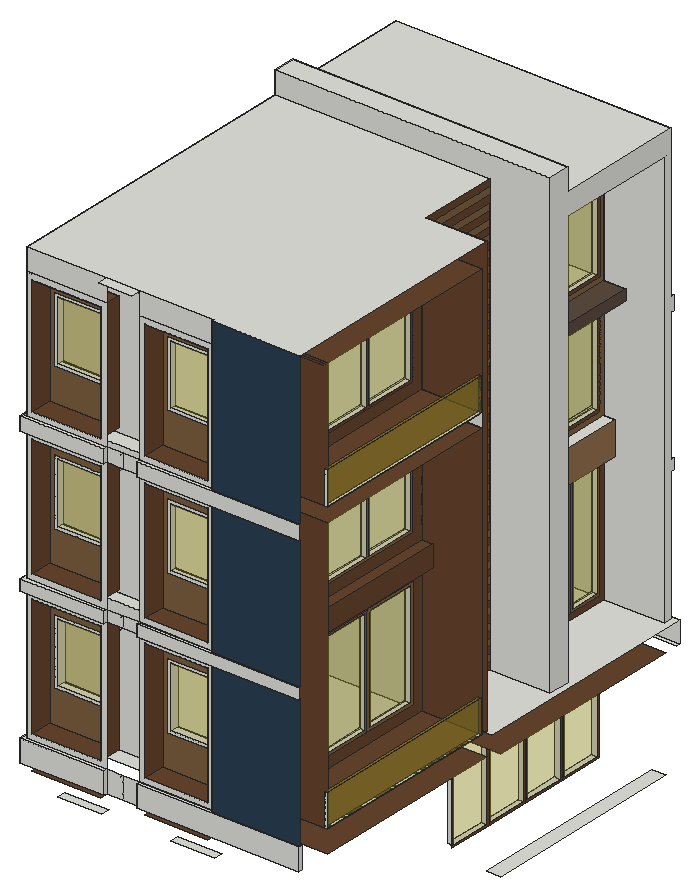
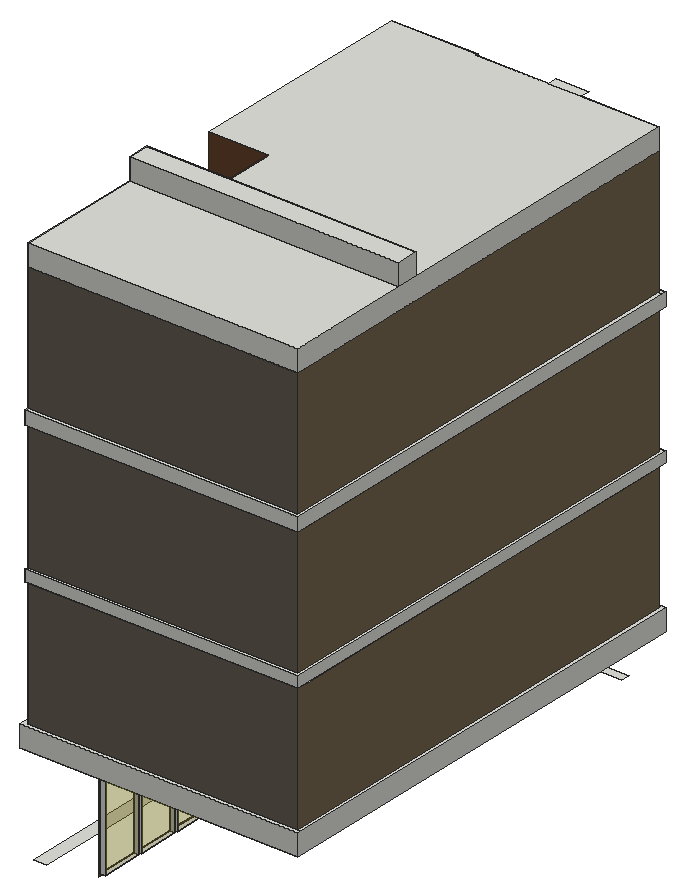
# SketchUp Ruby script. Lengths in inches.
U = 1.inch
M = Sketchup.active_model
def pt(a) = Geom::Point3d.new(a.map { |v| v * U })
def face(e, loops, mat)
  f = e.add_face(loops[0].map { |a| pt(a) })
  loops[1..].each { |l| e.add_face(l.map { |a| pt(a) }).erase! }
  f.material = f.back_material = mat if mat
  f
end
# faces: each face lists its corners as indices into pts; further lists are holes
def faces(e, pts, list, mat = nil) = list.each { |f| face(e, (f[0].is_a?(Array) ? f : [f]).map { |l| l.map { |i| pts[i] } }, mat) }
# xy, xz, yz: faces in a plane at the given z, y or x. An outline is a flat list of corners, or four numbers for a rectangle; further outlines are holes
def ring(l) = l.size == 4 ? [[l[0], l[1]], [l[2], l[1]], [l[2], l[3]], [l[0], l[3]]] : l.each_slice(2).to_a
def flat(e, list, mat, &to3) = list.each { |f| face(e, (f[0].is_a?(Array) ? f : [f]).map { |l| ring(l).map { |u, v| to3.(u, v) } }, mat) }
def xy(e, z, list, mat = nil) = flat(e, list, mat) { |x, y| [x, y, z] }
def xz(e, y, list, mat = nil) = flat(e, list, mat) { |x, z| [x, y, z] }
def yz(e, x, list, mat = nil) = flat(e, list, mat) { |y, z| [x, y, z] }
def lines(e, pts, list) = list.each { |a, b| e.add_line(pt(pts[a]), pt(pts[b])) }
# prism: a flat outline (further loops are holes) pulled along v
def prism(e, loops, v, mat = nil)
  f = face(e, loops, mat); d = Geom::Vector3d.new(v.map { |x| x * U })
  f.pushpull(f.normal.samedirection?(d) ? d.length : -d.length)
end
def box(e, o, s, mat = nil) = prism(e, [[o, [o[0] + s[0], o[1], o[2]], [o[0] + s[0], o[1] + s[1], o[2]], [o[0], o[1] + s[1], o[2]]]], [0, 0, s[2]], mat)
def at(x, y, z, deg = 0) = Geom::Transformation.translation(pt([x, y, z])) * Geom::Transformation.rotation(ORIGIN, Z_AXIS, deg.degrees)
def axes(o, x, y, z) = Geom::Transformation.new([*x, 0, *y, 0, *z, 0, *pt(o).to_a, 1])
def part(name) = M.definitions.add(name)
# library, detail: a bought-in or finely detailed component or shape, given as its bounding box
def library(name, o, s) = part(name).tap { |d| box(d.entities, o, s) }
def detail(e, o, s) = box(e.add_group.entities, o, s)
def put(e, d, t, mat = nil) = e.add_instance(d, t).tap { |i| i.material = mat if mat }
def group(e, t, mat = nil) = e.add_group.tap { |g| g.transformation = t; g.material = mat if mat }.entities
root = M.entities
M.materials.add("Carpet_04_1K").color = [43, 65, 85]
M.materials.add("Glass_Basic_01").color = [186, 175, 42]
M.materials["Glass_Basic_01"].alpha = 0.25
M.materials.add("Glass_Basic_1").color = [186, 174, 38]
M.materials["Glass_Basic_1"].alpha = 0.25
M.materials.add("Plaster_03_1K").color = [121, 105, 83]
M.materials.add("Plaster_04_1K").color = [106, 98, 87]
M.materials.add("Plywood_01_1K").color = [125, 96, 64]
M.materials.add("Wood_Floor_01_1K").color = [146, 111, 76]
M.materials.add("Wood_Floor_12_1K").color = [92, 75, 65]
M.materials.add("Wood_Veneer_15_1K").color = [103, 69, 45]
c1 = part("Group\#1")
xy(c1.entities,0,[[0,0,3,210]])
xy(c1.entities,36,[[0,0,3,210]],"Glass_Basic_01")
xz(c1.entities,0,[[0,0,3,36]])
xz(c1.entities,210,[[0,0,3,36]])
yz(c1.entities,0,[[0,0,210,36]],"Glass_Basic_01")
yz(c1.entities,3,[[0,0,210,36]],"Glass_Basic_01")
c2 = library("Sphere Light\#3",[-2.79,-2.79,-2.79],[5.58,5.58,5.58])
c3 = library("Sphere Light\#2",[-2.6,-2.6,-2.6],[5.2,5.2,5.2])
c4 = library("Sphere Light\#1",[-1.86,-1.86,-1.86],[3.72,3.72,3.72])
c5 = library("Sphere Light",[-2.55,-2.55,-2.55],[5.1,5.1,5.1])
xy(root,60,[[295,274,310,499]])
xy(root,62,[[241,288,247,334.25],[241,338.25,247,384.5],[241,388.5,247,434.75],[241,438.75,247,485]])
xy(root,141,[[19,34,67,43],[142,34,190,43]])
xy(root,165,[[241,49,247,119],[241,122,247,186],[241,189,247,259]])
xy(root,166,[[241,288,247,334.25],[241,338.25,247,384.5],[241,388.5,247,434.75],[241,438.75,247,485]])
xy(root,174,[[10,10,85,34],[133,10,202,34]],"Wood_Veneer_15_1K")
xy(root,180,[[0,6,4,514],[4,6,91,10],[127,6,127,10,208,10,208,8,304,8,304,6],[0,514,310,518]])
xy(root,180,[[208,8,304,10]],"Carpet_04_1K")
xy(root,180,[[247,46,304,262],[247,274,310,499]],"Wood_Veneer_15_1K")
xy(root,192,[[13,43,241,505]])
xy(root,204,[[0,6,4,514],[4,6,91,10],[127,6,304,6,304,8,208,8,208,10,127,10],[13,43,232,256],[238,262,310,262,310,518,0,518,0,514,304,514,304,505,238,505,238,373,304,373,304,349,238,349],
  [13,262,232,505]])
xy(root,204,[[208,8,304,10]],"Carpet_04_1K")
xy(root,204,[[238,46,304,256]],"Wood_Veneer_15_1K")
xy(root,210,[[10,10,85,34],[133,10,202,34]],"Wood_Veneer_15_1K")
xy(root,213,[[232,382,238,416],[232,422,238,456],[232,462,238,496]])
xy(root,219,[[232,61,238,117],[232,123,238,179],[232,185,238,241]])
xy(root,249,[[19,34,73,43],[142,34,196,43]])
xy(root,315,[[19,34,73,43],[142,34,196,43]])
xy(root,333,[[232,61,238,117],[232,123,238,179],[232,185,238,241]])
xy(root,339,[[232,382,238,416],[232,422,238,456],[232,462,238,496]])
xy(root,342,[[10,10,85,34],[133,10,202,34]],"Wood_Veneer_15_1K")
xy(root,348,[[0,6,4,43],[4,6,91,10],[127,6,127,10,208,10,208,8,304,8,304,6],[0,43,4,256],[4,43,13,256],
  [13,43,232,256],[0,256,4,262],[4,256,232,262],[0,262,4,349],[4,262,13,349],
  [13,262,232,505],[0,349,4,373],[4,349,13,373],[238,361,250,373],[0,373,4,505],
  [4,373,13,505],[238,373,250,505],[0,505,4,518],[4,514,304,518]])
xy(root,348,[[238,46,250,256]],"Wood_Veneer_15_1K")
xy(root,360,[[0,6,91,6,91,10,4,10,4,514,304,514,304,518,0,518],[127,6,304,6,304,8,208,8,208,10,127,10],[10,40,232,508]])
xy(root,366,[[10,10,85,34],[133,10,202,34]],"Wood_Veneer_15_1K")
xy(root,372,[[238,361,250,373]])
xy(root,372,[[238,46,250,256]],"Wood_Veneer_15_1K")
xy(root,384,[[238,373,250,505]])
xy(root,387,[[232,61,238,121],[232,124,238,181],[232,184,238,241]])
xy(root,393,[[232,382,238,436],[232,442,238,496]])
xy(root,405,[[19,34,73,40],[142,34,196,40]])
xy(root,471,[[19,34,73,40],[142,34,196,40]])
xy(root,489,[[232,61,238,121],[232,124,238,181],[232,184,238,241]])
xy(root,495,[[232,382,238,436],[232,442,238,496]])
xy(root,498,[[10,10,85,34],[133,10,202,34]],"Wood_Veneer_15_1K")
xy(root,504,[[0,6,91,10],[127,6,127,10,208,10,208,8,304,8,304,6],[0,10,4,508],[10,40,232,508],[232,43,238,46],
  [238,361,262,373],[0,508,4,518],[4,508,238,514],[4,514,238,518],[238,514,304,518]])
xy(root,504,[[238,373,262,505]],"Wood_Floor_12_1K")
xy(root,504,[[[238,46,304,256],[269.9,73.71,270.68,73.8125,271.4,74.11,272.02,74.59,272.5,75.21,272.8,75.93,272.9,76.71,272.8,77.49,272.5,78.21,272.02,78.83,271.4,79.31,270.68,79.61,269.9,79.71,269.125,79.61,268.4,79.31,267.78,78.83,267.3,78.21,267,77.49,266.9,76.71,267,75.93,267.3,75.21,267.78,74.59,268.4,74.11,269.125,73.8125],[269.9,225.375,270.68,225.48,271.4,225.78,272.02,226.26,272.5,226.875,272.8,227.6,272.9,228.375,272.8,229.15,272.5,229.875,272.02,230.5,271.4,230.97,270.68,231.27,269.9,231.375,269.125,231.27,268.4,230.97,267.78,230.5,267.3,229.875,267,229.15,266.9,228.375,267,227.6,267.3,226.875,267.78,226.26,268.4,225.78,269.125,225.48]]],"Wood_Veneer_15_1K")
xy(root,508,[[269.9,73.71,269.125,73.8125,268.4,74.11,267.78,74.59,267.3,75.21,267,75.93,266.9,76.71,267,77.49,267.3,78.21,267.78,78.83,268.4,79.31,269.125,79.61,269.9,79.71,270.68,79.61,271.4,79.31,272.02,78.83,272.5,78.21,272.8,77.49,272.9,76.71,272.8,75.93,272.5,75.21,272.02,74.59,271.4,74.11,270.68,73.8125],[269.9,225.375,269.125,225.48,268.4,225.78,267.78,226.26,267.3,226.875,267,227.6,266.9,228.375,267,229.15,267.3,229.875,267.78,230.5,268.4,230.97,269.125,231.27,269.9,231.375,270.68,231.27,271.4,230.97,272.02,230.5,272.5,229.875,272.8,229.15,272.9,228.375,272.8,227.6,272.5,226.875,272.02,226.26,271.4,225.78,270.68,225.48]],"Wood_Veneer_15_1K")
xy(root,516,[[10,40,232,508],[238,361,262,373]])
xy(root,516,[[238,373,262,505]],"Wood_Floor_12_1K")
xy(root,519,[[0,6,91,10],[127,6,304,6,304,8,208,8,208,10,127,10],[0,10,4,518],[4,514,304,518]])
xy(root,519,[[238,46,304,256]],"Wood_Veneer_15_1K")
xy(root,525,[[232,382,238,436],[232,442,238,496]])
xy(root,525,[[10,10,85,34],[133,10,202,34]],"Wood_Veneer_15_1K")
xy(root,534,[[232,61,238,121],[232,124,238,181],[232,184,238,241]])
xy(root,564,[[19,34,73,40],[142,34,196,40]])
xy(root,627,[[232,382,238,436],[232,442,238,496]])
xy(root,630,[[19,34,73,40],[142,34,196,40]])
xy(root,645,[[232,61,238,121],[232,124,238,181],[232,184,238,241]])
xy(root,654,[[10,10,85,34],[133,10,202,34]],"Wood_Veneer_15_1K")
xy(root,660,[[4,10,10,514],[10,40,232,508],[232,43,238,46],[232,46,238,262],[232,262,238,349],
  [232,349,238,508],[10,508,238,514]])
xy(root,660,[[[238,46,304,256],[269.9,73.71,270.68,73.8125,271.4,74.11,272.02,74.59,272.5,75.21,272.8,75.93,272.9,76.71,272.8,77.49,272.5,78.21,272.02,78.83,271.4,79.31,270.68,79.61,269.9,79.71,269.125,79.61,268.4,79.31,267.78,78.83,267.3,78.21,267,77.49,266.9,76.71,267,75.93,267.3,75.21,267.78,74.59,268.4,74.11,269.125,73.8125],[269.9,225.375,270.68,225.48,271.4,225.78,272.02,226.26,272.5,226.875,272.8,227.6,272.9,228.375,272.8,229.15,272.5,229.875,272.02,230.5,271.4,230.97,270.68,231.27,269.9,231.375,269.125,231.27,268.4,230.97,267.78,230.5,267.3,229.875,267,229.15,266.9,228.375,267,227.6,267.3,226.875,267.78,226.26,268.4,225.78,269.125,225.48]],[238,373,304,505]],"Wood_Veneer_15_1K")
xy(root,664,[[269.9,73.71,269.125,73.8125,268.4,74.11,267.78,74.59,267.3,75.21,267,75.93,266.9,76.71,267,77.49,267.3,78.21,267.78,78.83,268.4,79.31,269.125,79.61,269.9,79.71,270.68,79.61,271.4,79.31,272.02,78.83,272.5,78.21,272.8,77.49,272.9,76.71,272.8,75.93,272.5,75.21,272.02,74.59,271.4,74.11,270.68,73.8125],[269.9,225.375,269.125,225.48,268.4,225.78,267.78,226.26,267.3,226.875,267,227.6,266.9,228.375,267,229.15,267.3,229.875,267.78,230.5,268.4,230.97,269.125,231.27,269.9,231.375,270.68,231.27,271.4,230.97,272.02,230.5,272.5,229.875,272.8,229.15,272.9,228.375,272.8,227.6,272.5,226.875,272.02,226.26,271.4,225.78,270.68,225.48]],"Wood_Veneer_15_1K")
xy(root,684,[[91,0,127,10],[208,8,304,8,304,262,238,262,238,349,4,349,4,10,208,10],[4,373,304,514]])
xy(root,708,[[4,349,304,373]])
xz(root,6,[[0,180,91,204],[127,180,304,204],[0,348,91,360],[127,348,304,360],[0,504,91,519],
  [127,504,304,519]])
xz(root,8,[[208,204,304,348],[208,360,304,504],[208,519,304,684]],"Carpet_04_1K")
xz(root,10,[[91,180,109,204],[109,180,127,204],[127,180,208,204],[208,180,304,204],[[4,204,91,348],[10,210,85,342]],
  [[127,204,208,348],[133,210,202,342]],[91,348,109,360],[109,348,127,360],[127,348,208,360],[[4,360,91,504],[10,366,85,498]],
  [[127,360,208,504],[133,366,202,498]],[91,504,109,519],[109,504,127,519],[127,504,208,519],[[4,519,91,660],[10,525,85,654]],
  [[127,519,208,660],[133,525,202,654]],[4,660,91,684],[127,660,208,684]])
xz(root,34,[[[16,246,76,318],[19,249,73,315]],[[139,246,199,318],[142,249,196,315]],[[16,402,76,474],[19,405,73,471]],[[139,402,199,474],[142,405,196,471]],[[16,561,76,633],[19,564,73,630]],
  [[139,561,199,633],[142,564,196,630]]])
xz(root,34,[[19,249,73,315],[142,249,196,315],[19,405,73,471],[142,405,196,471],[19,564,73,630],
  [142,564,196,630]],"Glass_Basic_1")
xz(root,34,[[[10,210,85,342],[16,246,76,318]],[[133,210,202,342],[139,246,199,318]],[[10,366,85,498],[16,402,76,474]],[[133,366,202,498],[139,402,199,474]],[[10,525,85,654],[16,561,76,633]],
  [[133,525,202,654],[139,561,199,633]]],"Plywood_01_1K")
xz(root,40,[[[10,360,232,504],[19,405,73,471],[142,405,196,471]],[[10,516,232,660],[19,564,73,630],[142,564,196,630]]])
xz(root,40,[[19,405,73,471],[142,405,196,471],[19,564,73,630],[142,564,196,630]],"Glass_Basic_1")
xz(root,43,[[[13,204,232,348],[142,249,196,315],[19,249,73,315]]])
xz(root,43,[[19,249,73,315],[142,249,196,315]],"Glass_Basic_1")
xz(root,46,[[238,348,250,372]])
xz(root,46,[[238,204,238,348,250,348,250,372,238,372,238,504,304,504,304,240,301,240,301,204],[238,519,304,660]],"Wood_Veneer_15_1K")
xz(root,61,[[232,219,238,333],[232,387,238,489],[232,534,238,645]])
xz(root,117,[[232,219,238,333]])
xz(root,121,[[232,387,238,489],[232,534,238,645]])
xz(root,123,[[232,219,238,333]])
xz(root,124,[[232,387,238,489],[232,534,238,645]])
xz(root,179,[[232,219,238,333]])
xz(root,181,[[232,387,238,489],[232,534,238,645]])
xz(root,184,[[232,387,238,489],[232,534,238,645]])
xz(root,185,[[232,219,238,333]])
xz(root,241,[[232,219,238,333],[232,387,238,489],[232,534,238,645]])
xz(root,256,[[13,204,232,348],[238,348,250,360],[238,360,250,372],[238,504,304,519]])
xz(root,256,[[238,204,304,204,304,504,238,504,238,372,250,372,250,348,238,348],[238,519,304,660]],"Wood_Veneer_15_1K")
xz(root,262,[[13,204,232,348]])
xz(root,262,[[238,204,304,684]],"Wood_Veneer_15_1K")
xz(root,288,[[241,62,247,166]])
xz(root,334.25,[[241,62,247,166]])
xz(root,338.25,[[241,62,247,166]])
xz(root,349,[[238,204,304,204,304,708,4,708,4,684,238,684]])
xz(root,361,[[238,348,250,360],[238,360,250,372],[238,504,262,516]])
xz(root,373,[[238,372,250,384],[4,684,304,708]])
xz(root,373,[[238,204,238,348,250,348,250,384,238,384,238,504,262,504,262,516,238,516,238,660,304,660,304,204]],"Wood_Veneer_15_1K")
xz(root,382,[[232,213,238,339],[232,393,238,495],[232,525,238,627]])
xz(root,384.5,[[241,62,247,166]])
xz(root,388.5,[[241,62,247,166]])
xz(root,416,[[232,213,238,339]])
xz(root,422,[[232,213,238,339]])
xz(root,434.75,[[241,62,247,166]])
xz(root,436,[[232,393,238,495],[232,525,238,627]])
xz(root,438.75,[[241,62,247,166]])
xz(root,442,[[232,393,238,495],[232,525,238,627]])
xz(root,456,[[232,213,238,339]])
xz(root,462,[[232,213,238,339]])
xz(root,485,[[241,62,247,166]])
xz(root,496,[[232,213,238,339],[232,393,238,495],[232,525,238,627]])
xz(root,505,[[13,204,232,348],[238,204,304,204,304,660,238,660,238,516,262,516,262,504,238,504,238,384,250,384,250,348,238,348],[238,348,250,360],[238,360,250,384],[238,504,262,516]])
xz(root,508,[[10,360,232,504],[10,516,232,660]])
xz(root,514,[[4,660,304,684]])
xz(root,514,[[4,204,304,348],[4,360,304,504],[4,519,304,660]],"Plaster_04_1K")
xz(root,518,[[0,180,310,204],[0,348,304,360],[0,504,304,519]])
yz(root,0,[[6,180,518,204],[6,348,518,360],[6,504,518,519]])
yz(root,4,[[10,660,514,684],[349,684,373,708]])
yz(root,4,[[10,204,514,348],[10,360,514,504],[10,519,514,660]],"Plaster_03_1K")
yz(root,10,[[40,360,508,504],[40,516,508,660]])
yz(root,10,[[10,210,34,342],[10,366,34,498],[10,525,34,654]],"Wood_Veneer_15_1K")
yz(root,13,[[43,204,256,348],[262,204,505,348]])
yz(root,19,[[34,249,43,315],[34,405,40,471],[34,564,40,630]])
yz(root,73,[[34,249,43,315],[34,405,40,471],[34,564,40,630]])
yz(root,85,[[10,210,34,342],[10,366,34,498],[10,525,34,654]],"Wood_Veneer_15_1K")
yz(root,91,[[6,180,10,204],[6,348,10,360],[6,504,10,519]])
yz(root,127,[[6,180,10,204],[6,348,10,360],[6,504,10,519]])
yz(root,133,[[10,210,34,342],[10,366,34,498],[10,525,34,654]],"Wood_Veneer_15_1K")
yz(root,142,[[34,249,43,315],[34,405,40,471],[34,564,40,630]])
yz(root,196,[[34,249,43,315],[34,405,40,471],[34,564,40,630]])
yz(root,202,[[10,210,34,342],[10,366,34,498],[10,525,34,654]],"Wood_Veneer_15_1K")
yz(root,208,[[8,204,10,348],[8,360,10,504]],"Carpet_04_1K")
yz(root,208,[[8,519,10,660],[8,660,10,684]],"Plaster_04_1K")
yz(root,232,[[[43,204,256,348],[185,219,241,333],[123,219,179,333],[61,219,117,333]],[[262,204,505,348],[382,213,416,339],[422,213,456,339],[462,213,496,339]],[40,360,43,504],[43,360,46,504],[[46,360,508,504],[61,387,121,489],[184,387,241,489],[124,387,181,489],[442,393,496,495],[382,393,436,495]],
  [442,393,496,395.46],[40,516,43,660],[43,516,46,660],[[46,516,508,660],[61,534,121,645],[124,534,181,645],[184,534,241,645],[382,525,436,627],[442,525,496,627]]])
yz(root,232,[[382,213,416,339],[422,213,456,339],[462,213,496,339],[61,219,117,333],[123,219,179,333],
  [185,219,241,333],[61,387,121,489],[124,387,181,489],[184,387,241,489],[382,393,436,495],
  [442,395.46,496,495],[382,525,436,627],[442,525,496,627],[61,534,121,645],[124,534,181,645],
  [184,534,241,645]],"Glass_Basic_01")
yz(root,238,[[43,348,46,504],[256,348,262,360],[349,348,361,360],[256,360,262,504],[349,360,361,360,361,372,373,372,373,504,349,504],
  [43,504,46,660],[256,504,262,516],[349,504,361,516],[505,504,508,516],[256,516,262,660],
  [349,516,373,660],[505,516,508,660]])
yz(root,238,[[382,213,416,339],[422,213,456,339],[462,213,496,339],[61,219,117,333],[123,219,179,333],
  [185,219,241,333],[61,387,121,489],[124,387,181,489],[184,387,241,489],[382,393,436,495],
  [442,393,496,495],[382,525,436,627],[442,525,496,627],[61,534,121,645],[124,534,181,645],
  [184,534,241,645]],"Glass_Basic_01")
yz(root,238,[[[379,210,419,342],[382,213,416,339]],[[419,210,459,342],[422,213,456,339]],[[459,210,499,342],[462,213,496,339]],[262,211.6,349,219.2],[[58,216,120,336],[61,219,117,333]],
  [[120,216,182,336],[123,219,179,333]],[[182,216,244,336],[185,219,241,333]],[262,226.8,349,234.4],[262,242,349,249.6],[262,257.2,349,264.8],
  [262,272.4,349,280],[262,287.6,349,295.2],[262,302.8,349,310.4],[262,318,349,325.6],[262,333.2,349,340.8],
  [262,348.4,349,356],[262,363.6,349,371.2],[262,378.8,349,386.4],[[58,384,244,492],[61,387,61,489,121,489,121,387,124,387,124,489,181,489,181,387,184,387,184,489,241,489,241,387]],[[373,384,505,504],[379,390,499,498]],
  [262,394,349,401.6],[262,409.2,349,416.8],[262,424.4,349,432],[262,439.6,349,447.2],[262,454.8,349,462.4],
  [262,470,349,477.6],[262,485.2,349,492.8],[262,500.4,349,508],[262,515.6,349,523.2],[[373,516,505,636],[379,522,499,630]],
  [262,530.8,349,538.4],[262,546,349,553.6],[262,561.2,349,568.8],[262,576.4,349,584],[262,591.6,349,599.2],
  [262,606.8,349,614.4],[262,622,349,629.6],[262,637.2,349,644.8],[262,652.4,349,660],[262,668,349,676]],"Plywood_01_1K")
yz(root,238,[[373,636,505,660]],"Wood_Floor_01_1K")
yz(root,238,[[[46,204,256,348],[58,216,244,336]],[262,204,349,211.6],[[373,204,505,348],[379,210,499,342]],[262,219.2,349,226.8],[262,234.4,349,242],
  [262,249.6,349,257.2],[262,264.8,349,272.4],[262,280,349,287.6],[262,295.2,349,302.8],[262,310.4,349,318],
  [262,325.6,349,333.2],[262,340.8,349,348.4],[262,356,349,363.6],[262,371.2,349,378.8],[[46,372,256,504],[58,384,244,492]],
  [262,386.4,349,394],[[379,390,439,498],[382,393,436,495]],[[439,390,499,498],[442,393,496,495]],[262,401.6,349,409.2],[262,416.8,349,424.4],
  [262,432,349,439.6],[262,447.2,349,454.8],[262,462.4,349,470],[262,477.6,349,485.2],[262,492.8,349,500.4],
  [262,508,349,515.6],[[46,519,256,660],[58,531,244,648]],[[379,522,439,630],[382,525,436,627]],[[439,522,499,630],[442,525,496,627]],[262,523.2,349,530.8],
  [[58,531,244,648],[61,534,61,645,121,645,121,534,124,534,124,645,181,645,181,534,184,534,184,645,241,645,241,534]],[262,538.4,349,546],[262,553.6,349,561.2],[262,568.8,349,576.4],[262,584,349,591.6],
  [262,599.2,349,606.8],[262,614.4,349,622],[262,629.6,349,637.2],[262,644.8,349,652.4],[262,660,349,668],
  [262,676,349,684]],"Wood_Veneer_15_1K")
yz(root,241,[[288,62,334.25,166],[338.25,62,384.5,166],[388.5,62,434.75,166],[438.75,62,485,166]],"Glass_Basic_01")
yz(root,247,[[288,62,334.25,166],[338.25,62,384.5,166],[388.5,62,434.75,166],[438.75,62,485,166]],"Glass_Basic_01")
yz(root,247,[[[286,60,336.25,168],[288,62,334.25,166]],[[336.25,60,386.5,168],[338.25,62,384.5,166]],[[386.5,60,436.75,168],[388.5,62,434.75,166]],[[436.75,60,487,168],[438.75,62,485,166]]],"Wood_Veneer_15_1K")
yz(root,250,[[361,348,373,360],[361,360,373,372]])
yz(root,250,[[373,348,505,384]],"Wood_Floor_01_1K")
yz(root,250,[[46,348,256,372]],"Wood_Veneer_15_1K")
yz(root,262,[[361,504,373,516]])
yz(root,262,[[373,504,505,516]],"Wood_Floor_12_1K")
yz(root,304,[[6,180,10,204],[349,204,373,204,373,660,505,660,505,204,514,204,514,348,518,348,518,360,514,360,514,504,518,504,518,519,514,519,514,684,373,684,373,708,349,708]])
p = [[269.9,73.71,504],[269.125,73.8125,504],[269.125,73.8125,508],[269.9,73.71,508],[270.68,73.8125,504],[270.68,73.8125,508],
  [268.4,74.11,504],[268.4,74.11,508],[271.4,74.11,504],[271.4,74.11,508],[267.78,74.59,504],[267.78,74.59,508],
  [272.02,74.59,504],[272.02,74.59,508],[267.3,75.21,504],[267.3,75.21,508],[272.5,75.21,504],[272.5,75.21,508],
  [267,75.93,504],[267,75.93,508],[272.8,75.93,504],[272.8,75.93,508],[266.9,76.71,504],[266.9,76.71,508],
  [272.9,76.71,504],[272.9,76.71,508],[267,77.49,504],[267,77.49,508],[272.8,77.49,504],[272.8,77.49,508],
  [267.3,78.21,504],[267.3,78.21,508],[272.5,78.21,504],[272.5,78.21,508],[267.78,78.83,504],[267.78,78.83,508],
  [272.02,78.83,504],[272.02,78.83,508],[268.4,79.31,504],[268.4,79.31,508],[271.4,79.31,504],[271.4,79.31,508],
  [269.125,79.61,504],[269.125,79.61,508],[270.68,79.61,504],[270.68,79.61,508],[269.9,79.71,504],[269.9,79.71,508],
  [269.9,225.375,504],[269.125,225.48,504],[269.125,225.48,508],[269.9,225.375,508],[270.68,225.48,504],[270.68,225.48,508],
  [268.4,225.78,504],[268.4,225.78,508],[271.4,225.78,504],[271.4,225.78,508],[267.78,226.26,504],[267.78,226.26,508],
  [272.02,226.26,504],[272.02,226.26,508],[267.3,226.875,504],[267.3,226.875,508],[272.5,226.875,504],[272.5,226.875,508],
  [267,227.6,504],[267,227.6,508],[272.8,227.6,504],[272.8,227.6,508],[266.9,228.375,504],[266.9,228.375,508],
  [272.9,228.375,504],[272.9,228.375,508],[267,229.15,504],[267,229.15,508],[272.8,229.15,504],[272.8,229.15,508],
  [267.3,229.875,504],[267.3,229.875,508],[272.5,229.875,504],[272.5,229.875,508],[267.78,230.5,504],[267.78,230.5,508],
  [272.02,230.5,504],[272.02,230.5,508],[268.4,230.97,504],[268.4,230.97,508],[271.4,230.97,504],[271.4,230.97,508],
  [269.125,231.27,504],[269.125,231.27,508],[270.68,231.27,504],[270.68,231.27,508],[269.9,231.375,504],[269.9,231.375,508],
  [269.9,73.71,660],[269.125,73.8125,660],[269.125,73.8125,664],[269.9,73.71,664],[270.68,73.8125,660],[270.68,73.8125,664],
  [268.4,74.11,660],[268.4,74.11,664],[271.4,74.11,660],[271.4,74.11,664],[267.78,74.59,660],[267.78,74.59,664],
  [272.02,74.59,660],[272.02,74.59,664],[267.3,75.21,660],[267.3,75.21,664],[272.5,75.21,660],[272.5,75.21,664],
  [267,75.93,660],[267,75.93,664],[272.8,75.93,660],[272.8,75.93,664],[266.9,76.71,660],[266.9,76.71,664],
  [272.9,76.71,660],[272.9,76.71,664],[267,77.49,660],[267,77.49,664],[272.8,77.49,660],[272.8,77.49,664],
  [267.3,78.21,660],[267.3,78.21,664],[272.5,78.21,660],[272.5,78.21,664],[267.78,78.83,660],[267.78,78.83,664],
  [272.02,78.83,660],[272.02,78.83,664],[268.4,79.31,660],[268.4,79.31,664],[271.4,79.31,660],[271.4,79.31,664],
  [269.125,79.61,660],[269.125,79.61,664],[270.68,79.61,660],[270.68,79.61,664],[269.9,79.71,660],[269.9,79.71,664],
  [269.9,225.375,660],[269.125,225.48,660],[269.125,225.48,664],[269.9,225.375,664],[270.68,225.48,660],[270.68,225.48,664],
  [268.4,225.78,660],[268.4,225.78,664],[271.4,225.78,660],[271.4,225.78,664],[267.78,226.26,660],[267.78,226.26,664],
  [272.02,226.26,660],[272.02,226.26,664],[267.3,226.875,660],[267.3,226.875,664],[272.5,226.875,660],[272.5,226.875,664],
  [267,227.6,660],[267,227.6,664],[272.8,227.6,660],[272.8,227.6,664],[266.9,228.375,660],[266.9,228.375,664],
  [272.9,228.375,660],[272.9,228.375,664],[267,229.15,660],[267,229.15,664],[272.8,229.15,660],[272.8,229.15,664],
  [267.3,229.875,660],[267.3,229.875,664],[272.5,229.875,660],[272.5,229.875,664],[267.78,230.5,660],[267.78,230.5,664],
  [272.02,230.5,660],[272.02,230.5,664],[268.4,230.97,660],[268.4,230.97,664],[271.4,230.97,660],[271.4,230.97,664],
  [269.125,231.27,660],[269.125,231.27,664],[270.68,231.27,660],[270.68,231.27,664],[269.9,231.375,660],[269.9,231.375,664],
  [247,505,192],[247,514,192],[241,43,192],[247,43,192],[241,505,192],[232,43,348],
  [238,43,348],[238,34,348],[232,40,504],[232,34,504],[238,508,516],[238,514,516],
  [232,40,660],[304,40,660],[238,43,660],[304,43,660],[238,508,660],[304,508,660],
  [109,10,519],[109,6,519],[109,10,504],[109,6,504],[109,10,360],[109,6,360],
  [109,10,348],[109,6,348],[109,10,204],[109,6,204]]
faces(root,p,[[0,1,2,3],[4,0,3,5],[1,6,7,2],[8,4,5,9],[6,10,11,7],[12,8,9,13],[10,14,15,11],[16,12,13,17],
  [14,18,19,15],[20,16,17,21],[18,22,23,19],[24,20,21,25],[22,26,27,23],[28,24,25,29],[26,30,31,27],[32,28,29,33],
  [30,34,35,31],[36,32,33,37],[34,38,39,35],[40,36,37,41],[38,42,43,39],[44,40,41,45],[42,46,47,43],[46,44,45,47],
  [48,49,50,51],[52,48,51,53],[49,54,55,50],[56,52,53,57],[54,58,59,55],[60,56,57,61],[58,62,63,59],[64,60,61,65],
  [62,66,67,63],[68,64,65,69],[66,70,71,67],[72,68,69,73],[70,74,75,71],[76,72,73,77],[74,78,79,75],[80,76,77,81],
  [78,82,83,79],[84,80,81,85],[82,86,87,83],[88,84,85,89],[86,90,91,87],[92,88,89,93],[90,94,95,91],[94,92,93,95],
  [96,97,98,99],[100,96,99,101],[97,102,103,98],[104,100,101,105],[102,106,107,103],[108,104,105,109],[106,110,111,107],[112,108,109,113],
  [110,114,115,111],[116,112,113,117],[114,118,119,115],[120,116,117,121],[118,122,123,119],[124,120,121,125],[122,126,127,123],[128,124,125,129],
  [126,130,131,127],[132,128,129,133],[130,134,135,131],[136,132,133,137],[134,138,139,135],[140,136,137,141],[138,142,143,139],[142,140,141,143],
  [144,145,146,147],[148,144,147,149],[145,150,151,146],[152,148,149,153],[150,154,155,151],[156,152,153,157],[154,158,159,155],[160,156,157,161],
  [158,162,163,159],[164,160,161,165],[162,166,167,163],[168,164,165,169],[166,170,171,167],[172,168,169,173],[170,174,175,171],[176,172,173,177],
  [174,178,179,175],[180,176,177,181],[178,182,183,179],[184,180,181,185],[182,186,187,183],[188,184,185,189],[186,190,191,187],[190,188,189,191]],"Wood_Veneer_15_1K")
lines(root,p,[[192,193],[194,195],[196,192],[197,198],[199,198],[200,201],[202,203],[204,205],[206,207],[208,209],[210,211],[212,213],
  [214,215],[216,217],[218,219]])
put(root,c1,at(301,46,204))
put(root,c2,at(269.97,228.3,508))
put(root,c3,at(269.875,76.61,508))
put(root,c1,at(301,46,519))
put(root,c4,at(269.9,228.375,660))
put(root,c5,at(269.62,76.57,662.52))
